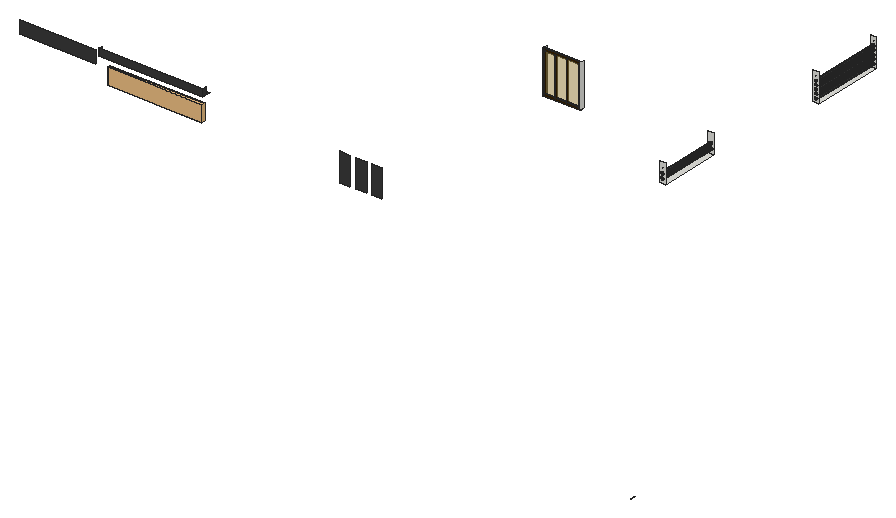
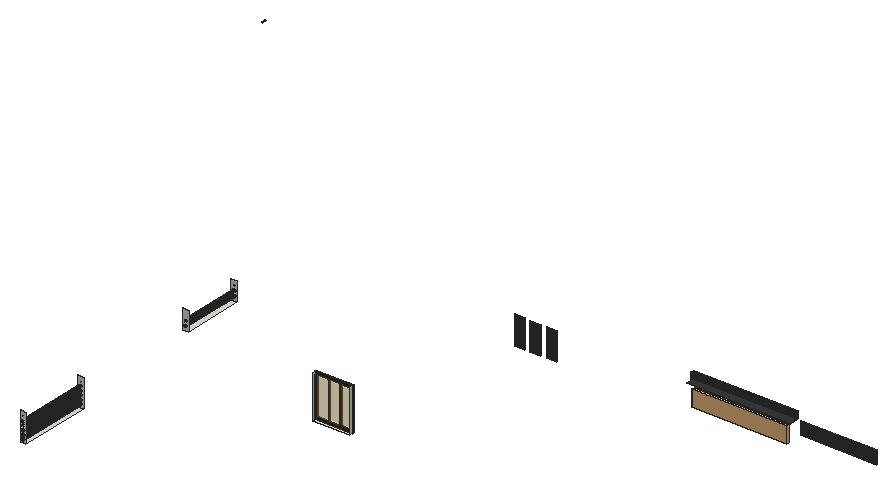
# SketchUp Ruby script. Lengths in inches.
U = 1.inch
M = Sketchup.active_model
def pt(a) = Geom::Point3d.new(a.map { |v| v * U })
def face(e, loops, mat)
  f = e.add_face(loops[0].map { |a| pt(a) })
  loops[1..].each { |l| e.add_face(l.map { |a| pt(a) }).erase! }
  f.material = f.back_material = mat if mat
  f
end
# faces: each face lists its corners as indices into pts; further lists are holes
def faces(e, pts, list, mat = nil) = list.each { |f| face(e, (f[0].is_a?(Array) ? f : [f]).map { |l| l.map { |i| pts[i] } }, mat) }
# xy, xz, yz: faces in a plane at the given z, y or x. An outline is a flat list of corners, or four numbers for a rectangle; further outlines are holes
def ring(l) = l.size == 4 ? [[l[0], l[1]], [l[2], l[1]], [l[2], l[3]], [l[0], l[3]]] : l.each_slice(2).to_a
def flat(e, list, mat, &to3) = list.each { |f| face(e, (f[0].is_a?(Array) ? f : [f]).map { |l| ring(l).map { |u, v| to3.(u, v) } }, mat) }
def xy(e, z, list, mat = nil) = flat(e, list, mat) { |x, y| [x, y, z] }
def xz(e, y, list, mat = nil) = flat(e, list, mat) { |x, z| [x, y, z] }
def yz(e, x, list, mat = nil) = flat(e, list, mat) { |y, z| [x, y, z] }
def lines(e, pts, list) = list.each { |a, b| e.add_line(pt(pts[a]), pt(pts[b])) }
# prism: a flat outline (further loops are holes) pulled along v
def prism(e, loops, v, mat = nil)
  f = face(e, loops, mat); d = Geom::Vector3d.new(v.map { |x| x * U })
  f.pushpull(f.normal.samedirection?(d) ? d.length : -d.length)
end
def box(e, o, s, mat = nil) = prism(e, [[o, [o[0] + s[0], o[1], o[2]], [o[0] + s[0], o[1] + s[1], o[2]], [o[0], o[1] + s[1], o[2]]]], [0, 0, s[2]], mat)
def at(x, y, z, deg = 0) = Geom::Transformation.translation(pt([x, y, z])) * Geom::Transformation.rotation(ORIGIN, Z_AXIS, deg.degrees)
def axes(o, x, y, z) = Geom::Transformation.new([*x, 0, *y, 0, *z, 0, *pt(o).to_a, 1])
def part(name) = M.definitions.add(name)
# library, detail: a bought-in or finely detailed component or shape, given as its bounding box
def library(name, o, s) = part(name).tap { |d| box(d.entities, o, s) }
def detail(e, o, s) = box(e.add_group.entities, o, s)
def put(e, d, t, mat = nil) = e.add_instance(d, t).tap { |i| i.material = mat if mat }
def group(e, t, mat = nil) = e.add_group.tap { |g| g.transformation = t; g.material = mat if mat }.entities
root = M.entities
M.materials.add("[Color A08]").color = [56, 34, 0]
M.materials.add("[Color M07]").color = [58, 58, 58]
M.materials.add("[Color M08]").color = [30, 30, 30]
M.materials.add("[Translucent Glass Blue]").color = [179, 149, 61]
M.materials["[Translucent Glass Blue]"].alpha = 0.5
c1 = part("Group\#2")
xy(c1.entities,0,[[0,0,80.25,5.625]],"[Color A08]")
xy(c1.entities,3.1,[[3.1,0,25.78,5.625],[27.03,0,50.28,5.625],[51.53,0,77.15,5.625]],"[Color A08]")
xy(c1.entities,66.65,[[3.1,0,25.78,5.625],[27.03,0,50.28,5.625],[51.53,0,77.15,5.625]],"[Color A08]")
xy(c1.entities,69.75,[[0,0,80.25,5.625]],"[Color A08]")
xz(c1.entities,0,[[[0,0,80.25,69.75],[51.53,3.1,77.15,66.65],[27.03,3.1,50.28,66.65],[3.1,3.1,25.78,66.65]]],"[Color A08]")
xz(c1.entities,5.625,[[[0,0,80.25,69.75],[51.53,3.1,77.15,66.65],[27.03,3.1,50.28,66.65],[3.1,3.1,25.78,66.65]]],"[Color A08]")
xz(c1.entities,5.625,[[3.1,3.1,25.78,66.65],[27.03,3.1,50.28,66.65],[51.53,3.1,77.15,66.65]],"[Translucent Glass Blue]")
yz(c1.entities,0,[[0,0,5.625,69.75]],"[Color A08]")
yz(c1.entities,3.1,[[0,3.1,5.625,66.65]],"[Color A08]")
yz(c1.entities,25.78,[[0,3.1,5.625,66.65]],"[Color A08]")
yz(c1.entities,27.03,[[0,3.1,5.625,66.65]],"[Color A08]")
yz(c1.entities,50.28,[[0,3.1,5.625,66.65]],"[Color A08]")
yz(c1.entities,51.53,[[0,3.1,5.625,66.65]],"[Color A08]")
yz(c1.entities,77.15,[[0,3.1,5.625,66.65]],"[Color A08]")
yz(c1.entities,80.25,[[0,0,5.625,69.75]],"[Color A08]")
c2 = library("Housedekho",[0.59,0,0],[171.25,24.51,4])
xy(root,58.07,[[560.85,700.96,616.42,706.96]])
xy(root,64.65,[[1254.01,0,1254.88,6]],"[Color M08]")
xy(root,70.51,[[831,872.22,840,980.28]])
xy(root,88.15,[[831,582.45,840,674.33]])
xy(root,94.09,[[132.5,398.15,288.93,411.21]],"[Color M07]")
xz(root,398.15,[[132.5,94.09,288.93,105]],"[Color M07]")
xz(root,402.9,[[491.76,47.23,507.7,89.6],[516.07,47.23,532.01,89.6],[540.01,47.23,555.95,89.6],[9.54,78.4,123.17,97.78]],"[Color M07]")
xz(root,582.45,[[[831,88.15,840,117.03],[835.26,93.06,835.76,93.07,836.25,93.21,836.68,93.48,837.03,93.84,837.27,94.29,837.39,94.78,837.38,95.28,837.23,95.77,836.97,96.2,836.61,96.55,836.16,96.79,835.67,96.91,835.16,96.9,834.68,96.76,834.25,96.49,833.9,96.13,833.66,95.68,833.54,95.19,833.55,94.6875,833.69,94.2,833.95,93.77,834.32,93.42,834.76,93.18],[835.13,100,835.64,100.01,836.12,100.15,836.55,100.41,836.9,100.78,837.14,101.22,837.26,101.71,837.25,102.22,837.11,102.71,836.85,103.14,836.48,103.49,836.04,103.73,835.55,103.85,835.04,103.84,834.55,103.69,834.12,103.43,833.77,103.06,833.53,102.62,833.41,102.13,833.42,101.625,833.57,101.14,833.83,100.71,834.19,100.36,834.64,100.11],[835.13,107.31,835.64,107.32,836.12,107.46,836.55,107.73,836.9,108.09,837.14,108.54,837.26,109.03,837.25,109.53,837.11,110.02,836.85,110.45,836.48,110.8,836.04,111.04,835.55,111.16,835.04,111.15,834.55,111.01,834.12,110.74,833.77,110.38,833.53,109.93,833.41,109.44,833.42,108.9375,833.57,108.45,833.83,108.02,834.19,107.67,834.64,107.43]]])
xz(root,582.45,[[835.26,93.06,835.76,93.07,836.25,93.21,836.68,93.48,837.03,93.84,837.27,94.29,837.39,94.78,837.38,95.28,837.23,95.77,836.97,96.2,836.61,96.55,836.16,96.79,835.67,96.91,835.16,96.9,834.68,96.76,834.25,96.49,833.9,96.13,833.66,95.68,833.54,95.19,833.55,94.6875,833.69,94.2,833.95,93.77,834.32,93.42,834.76,93.18],[835.13,100,835.64,100.01,836.12,100.15,836.55,100.41,836.9,100.78,837.14,101.22,837.26,101.71,837.25,102.22,837.11,102.71,836.85,103.14,836.48,103.49,836.04,103.73,835.55,103.85,835.04,103.84,834.55,103.69,834.12,103.43,833.77,103.06,833.53,102.62,833.41,102.13,833.42,101.625,833.57,101.14,833.83,100.71,834.19,100.36,834.64,100.11]],"[Color M07]")
xz(root,674.14,[[835.13,100,834.64,100.11,834.19,100.36,833.83,100.71,833.57,101.14,833.42,101.625,833.41,102.13,833.53,102.62,833.77,103.06,834.12,103.43,834.55,103.69,835.04,103.84,835.55,103.85,836.04,103.73,836.48,103.49,836.85,103.14,837.11,102.71,837.25,102.22,837.26,101.71,837.14,101.22,836.9,100.78,836.55,100.41,836.12,100.15,835.64,100.01]],"[Color M07]")
xz(root,674.2,[[835.26,93.06,834.76,93.18,834.32,93.42,833.95,93.77,833.69,94.2,833.55,94.6875,833.54,95.19,833.66,95.68,833.9,96.13,834.25,96.49,834.68,96.76,835.16,96.9,835.67,96.91,836.16,96.79,836.61,96.55,836.97,96.2,837.23,95.77,837.38,95.28,837.39,94.78,837.27,94.29,837.03,93.84,836.68,93.48,836.25,93.21,835.76,93.07]],"[Color M07]")
xz(root,674.33,[[831,88.15,840,117.03]])
xz(root,872.22,[[[831,70.51,840,113.38],[835.68,80.13,836.15,80.18,836.59,80.36,836.97,80.64,837.27,81.01,837.45,81.44,837.53,81.91,837.47,82.38,837.3,82.82,837.02,83.2,836.65,83.49,836.21,83.68,835.75,83.75,835.28,83.7,834.84,83.53,834.46,83.25,834.16,82.88,833.97,82.44,833.9,81.98,833.95,81.51,834.125,81.07,834.41,80.68,834.78,80.39,835.21,80.2],[835.68,86.19,836.15,86.25,836.59,86.42,836.97,86.7,837.27,87.07,837.45,87.5,837.53,87.97,837.47,88.44,837.3,88.88,837.02,89.26,836.65,89.56,836.21,89.75,835.75,89.82,835.28,89.76,834.84,89.59,834.46,89.31,834.16,88.94,833.97,88.51,833.9,88.04,833.95,87.57,834.125,87.13,834.41,86.75,834.78,86.45,835.21,86.26],[835.68,92.25,836.15,92.31,836.59,92.48,836.97,92.76,837.27,93.13,837.45,93.57,837.53,94.03,837.47,94.5,837.3,94.94,837.02,95.32,836.65,95.62,836.21,95.81,835.75,95.88,835.28,95.83,834.84,95.65,834.46,95.37,834.16,95,833.97,94.57,833.9,94.1,833.95,93.63,834.125,93.19,834.41,92.81,834.78,92.51,835.21,92.33],[835.68,98.32,836.15,98.37,836.59,98.54,836.97,98.82,837.27,99.19,837.45,99.63,837.53,100.1,837.47,100.57,837.3,101.01,837.02,101.39,836.65,101.68,836.21,101.87,835.75,101.94,835.28,101.89,834.84,101.72,834.46,101.43,834.16,101.06,833.97,100.63,833.9,100.16,833.95,99.69,834.125,99.25,834.41,98.87,834.78,98.58,835.21,98.39],[835.68,104.38,836.15,104.43,836.59,104.61,836.97,104.89,837.27,105.26,837.45,105.69,837.53,106.16,837.47,106.63,837.3,107.07,837.02,107.45,836.65,107.74,836.21,107.93,835.75,108,835.28,107.95,834.84,107.78,834.46,107.5,834.16,107.13,833.97,106.69,833.9,106.23,833.95,105.76,834.125,105.32,834.41,104.93,834.78,104.64,835.21,104.45],[835.68,74.07,836.15,74.12,836.59,74.29,836.97,74.57,837.27,74.94,837.45,75.38,837.53,75.85,837.47,76.32,837.3,76.76,837.02,77.14,836.65,77.43,836.21,77.62,835.75,77.69,835.28,77.64,834.84,77.47,834.46,77.18,834.16,76.81,833.97,76.38,833.9,75.91,833.95,75.44,834.125,75,834.41,74.62,834.78,74.33,835.21,74.14]]])
xz(root,872.22,[[835.68,74.07,836.15,74.12,836.59,74.29,836.97,74.57,837.27,74.94,837.45,75.38,837.53,75.85,837.47,76.32,837.3,76.76,837.02,77.14,836.65,77.43,836.21,77.62,835.75,77.69,835.28,77.64,834.84,77.47,834.46,77.18,834.16,76.81,833.97,76.38,833.9,75.91,833.95,75.44,834.125,75,834.41,74.62,834.78,74.33,835.21,74.14],[835.68,80.13,836.15,80.18,836.59,80.36,836.97,80.64,837.27,81.01,837.45,81.44,837.53,81.91,837.47,82.38,837.3,82.82,837.02,83.2,836.65,83.49,836.21,83.68,835.75,83.75,835.28,83.7,834.84,83.53,834.46,83.25,834.16,82.88,833.97,82.44,833.9,81.98,833.95,81.51,834.125,81.07,834.41,80.68,834.78,80.39,835.21,80.2],[835.68,86.19,836.15,86.25,836.59,86.42,836.97,86.7,837.27,87.07,837.45,87.5,837.53,87.97,837.47,88.44,837.3,88.88,837.02,89.26,836.65,89.56,836.21,89.75,835.75,89.82,835.28,89.76,834.84,89.59,834.46,89.31,834.16,88.94,833.97,88.51,833.9,88.04,833.95,87.57,834.125,87.13,834.41,86.75,834.78,86.45,835.21,86.26],[835.68,92.25,836.15,92.31,836.59,92.48,836.97,92.76,837.27,93.13,837.45,93.57,837.53,94.03,837.47,94.5,837.3,94.94,837.02,95.32,836.65,95.62,836.21,95.81,835.75,95.88,835.28,95.83,834.84,95.65,834.46,95.37,834.16,95,833.97,94.57,833.9,94.1,833.95,93.63,834.125,93.19,834.41,92.81,834.78,92.51,835.21,92.33],[835.68,98.32,836.15,98.37,836.59,98.54,836.97,98.82,837.27,99.19,837.45,99.63,837.53,100.1,837.47,100.57,837.3,101.01,837.02,101.39,836.65,101.68,836.21,101.87,835.75,101.94,835.28,101.89,834.84,101.72,834.46,101.43,834.16,101.06,833.97,100.63,833.9,100.16,833.95,99.69,834.125,99.25,834.41,98.87,834.78,98.58,835.21,98.39]],"[Color M07]")
xz(root,980.03,[[835.68,92.25,835.21,92.33,834.78,92.51,834.41,92.81,834.125,93.19,833.95,93.63,833.9,94.1,833.97,94.57,834.16,95,834.46,95.37,834.84,95.65,835.28,95.83,835.75,95.88,836.21,95.81,836.65,95.62,837.02,95.32,837.3,94.94,837.47,94.5,837.53,94.03,837.45,93.57,837.27,93.13,836.97,92.76,836.59,92.48,836.15,92.31],[835.68,98.32,835.21,98.39,834.78,98.58,834.41,98.87,834.125,99.25,833.95,99.69,833.9,100.16,833.97,100.63,834.16,101.06,834.46,101.43,834.84,101.72,835.28,101.89,835.75,101.94,836.21,101.87,836.65,101.68,837.02,101.39,837.3,101.01,837.47,100.57,837.53,100.1,837.45,99.63,837.27,99.19,836.97,98.82,836.59,98.54,836.15,98.37]],"[Color M07]")
xz(root,980.28,[[[831,70.51,840,113.38],[835.68,86.19,835.21,86.26,834.78,86.45,834.41,86.75,834.125,87.13,833.95,87.57,833.9,88.04,833.97,88.51,834.16,88.94,834.46,89.31,834.84,89.59,835.28,89.76,835.75,89.82,836.21,89.75,836.65,89.56,837.02,89.26,837.3,88.88,837.47,88.44,837.53,87.97,837.45,87.5,837.27,87.07,836.97,86.7,836.59,86.42,836.15,86.25],[835.68,104.38,835.21,104.45,834.78,104.64,834.41,104.93,834.125,105.32,833.95,105.76,833.9,106.23,833.97,106.69,834.16,107.13,834.46,107.5,834.84,107.78,835.28,107.95,835.75,108,836.21,107.93,836.65,107.74,837.02,107.45,837.3,107.07,837.47,106.63,837.53,106.16,837.45,105.69,837.27,105.26,836.97,104.89,836.59,104.61,836.15,104.43]]])
xz(root,980.34,[[835.68,74.07,835.21,74.14,834.78,74.33,834.41,74.62,834.125,75,833.95,75.44,833.9,75.91,833.97,76.38,834.16,76.81,834.46,77.18,834.84,77.47,835.28,77.64,835.75,77.69,836.21,77.62,836.65,77.43,837.02,77.14,837.3,76.76,837.47,76.32,837.53,75.85,837.45,75.38,837.27,74.94,836.97,74.57,836.59,74.29,836.15,74.12]],"[Color M07]")
xz(root,981.09,[[835.68,80.13,835.21,80.2,834.78,80.39,834.41,80.68,834.125,81.07,833.95,81.51,833.9,81.98,833.97,82.44,834.16,82.88,834.46,83.25,834.84,83.53,835.28,83.7,835.75,83.75,836.21,83.68,836.65,83.49,837.02,83.2,837.3,82.82,837.47,82.38,837.53,81.91,837.45,81.44,837.27,81.01,836.97,80.64,836.59,80.36,836.15,80.18]],"[Color M07]")
yz(root,132.5,[[398.15,94.09,402.9,105]],"[Color M07]")
yz(root,288.93,[[398.15,94.09,402.9,105]],"[Color M07]")
yz(root,560.85,[[700.96,58.07,706.96,122.82]])
yz(root,616.42,[[700.96,58.07,706.96,122.82]])
p = [[835.21,872.22,74.14],[834.78,872.22,74.33],[834.78,980.34,74.33],[835.21,980.34,74.14],[835.68,872.22,74.07],[835.68,980.34,74.07],
  [836.15,872.22,74.12],[836.15,980.34,74.12],[836.59,872.22,74.29],[836.59,980.34,74.29],[834.41,872.22,74.62],[834.41,980.34,74.62],
  [836.97,872.22,74.57],[836.97,980.34,74.57],[834.125,872.22,75],[834.125,980.34,75],[837.27,872.22,74.94],[837.27,980.34,74.94],
  [837.45,872.22,75.38],[837.45,980.34,75.38],[833.95,872.22,75.44],[833.95,980.34,75.44],[833.9,872.22,75.91],[833.9,980.34,75.91],
  [837.53,872.22,75.85],[837.53,980.34,75.85],[837.47,872.22,76.32],[837.47,980.34,76.32],[833.97,872.22,76.38],[833.97,980.34,76.38],
  [837.3,872.22,76.76],[837.3,980.34,76.76],[834.16,872.22,76.81],[834.16,980.34,76.81],[834.46,872.22,77.18],[834.46,980.34,77.18],
  [837.02,872.22,77.14],[837.02,980.34,77.14],[836.65,872.22,77.43],[836.65,980.34,77.43],[834.84,872.22,77.47],[834.84,980.34,77.47],
  [836.21,872.22,77.62],[836.21,980.34,77.62],[835.28,872.22,77.64],[835.28,980.34,77.64],[835.75,872.22,77.69],[835.75,980.34,77.69],
  [835.68,872.22,80.13],[835.21,872.22,80.2],[835.21,981.09,80.2],[835.68,981.09,80.13],[836.15,872.22,80.18],[836.15,981.09,80.18],
  [834.78,872.22,80.39],[834.78,981.09,80.39],[836.59,872.22,80.36],[836.59,981.09,80.36],[834.41,872.22,80.68],[834.41,981.09,80.68],
  [836.97,872.22,80.64],[836.97,981.09,80.64],[837.27,872.22,81.01],[837.27,981.09,81.01],[834.125,872.22,81.07],[834.125,981.09,81.07],
  [837.45,872.22,81.44],[837.45,981.09,81.44],[833.95,872.22,81.51],[833.95,981.09,81.51],[837.53,872.22,81.91],[837.53,981.09,81.91],
  [833.9,872.22,81.98],[833.9,981.09,81.98],[837.47,872.22,82.38],[837.47,981.09,82.38],[833.97,872.22,82.44],[833.97,981.09,82.44],
  [834.16,872.22,82.88],[834.16,981.09,82.88],[837.3,872.22,82.82],[837.3,981.09,82.82],[837.02,872.22,83.2],[837.02,981.09,83.2],
  [834.46,872.22,83.25],[834.46,981.09,83.25],[834.84,872.22,83.53],[834.84,981.09,83.53],[836.65,872.22,83.49],[836.65,981.09,83.49],
  [835.28,872.22,83.7],[835.28,981.09,83.7],[836.21,872.22,83.68],[836.21,981.09,83.68],[835.75,872.22,83.75],[835.75,981.09,83.75],
  [835.68,872.22,86.19],[835.21,872.22,86.26],[835.21,980.28,86.26],[835.68,980.28,86.19],[836.15,872.22,86.25],[836.15,980.28,86.25],
  [836.59,872.22,86.42],[836.59,980.28,86.42],[834.78,872.22,86.45],[834.78,980.28,86.45],[836.97,872.22,86.7],[836.97,980.28,86.7],
  [834.41,872.22,86.75],[834.41,980.28,86.75],[834.125,872.22,87.13],[834.125,980.28,87.13],[837.27,872.22,87.07],[837.27,980.28,87.07],
  [833.95,872.22,87.57],[833.95,980.28,87.57],[837.45,872.22,87.5],[837.45,980.28,87.5],[837.53,872.22,87.97],[837.53,980.28,87.97],
  [833.9,872.22,88.04],[833.9,980.28,88.04],[833.97,872.22,88.51],[833.97,980.28,88.51],[837.47,872.22,88.44],[837.47,980.28,88.44],
  [837.3,872.22,88.88],[837.3,980.28,88.88],[834.16,872.22,88.94],[834.16,980.28,88.94],[834.46,872.22,89.31],[834.46,980.28,89.31],
  [837.02,872.22,89.26],[837.02,980.28,89.26],[834.84,872.22,89.59],[834.84,980.28,89.59],[836.65,872.22,89.56],[836.65,980.28,89.56],
  [835.28,872.22,89.76],[835.28,980.28,89.76],[836.21,872.22,89.75],[836.21,980.28,89.75],[835.75,872.22,89.82],[835.75,980.28,89.82],
  [835.21,872.22,92.33],[834.78,872.22,92.51],[834.78,980.03,92.51],[835.21,980.03,92.33],[835.68,872.22,92.25],[835.68,980.03,92.25],
  [836.15,872.22,92.31],[836.15,980.03,92.31],[836.59,872.22,92.48],[836.59,980.03,92.48],[834.41,872.22,92.81],[834.41,980.03,92.81],
  [836.97,872.22,92.76],[836.97,980.03,92.76],[834.125,872.22,93.19],[834.125,980.03,93.19],[837.27,872.22,93.13],[837.27,980.03,93.13],
  [835.26,582.45,93.06],[834.76,582.45,93.18],[834.76,674.2,93.18],[835.26,674.2,93.06],[835.76,582.45,93.07],[835.76,674.2,93.07],
  [836.25,582.45,93.21],[836.25,674.2,93.21],[837.45,872.22,93.57],[837.45,980.03,93.57],[834.32,582.45,93.42],[834.32,674.2,93.42],
  [836.68,582.45,93.48],[836.68,674.2,93.48],[833.95,872.22,93.63],[833.95,980.03,93.63],[833.95,582.45,93.77],[833.95,674.2,93.77],
  [837.03,582.45,93.84],[837.03,674.2,93.84],[833.9,872.22,94.1],[833.9,980.03,94.1],[837.53,872.22,94.03],[837.53,980.03,94.03],
  [833.69,582.45,94.2],[833.69,674.2,94.2],[837.27,582.45,94.29],[837.27,674.2,94.29],[837.47,872.22,94.5],[837.47,980.03,94.5],
  [833.97,872.22,94.57],[833.97,980.03,94.57],[833.55,582.45,94.6875],[833.55,674.2,94.6875],[837.39,582.45,94.78],[837.39,674.2,94.78],
  [837.3,872.22,94.94],[837.3,980.03,94.94],[834.16,872.22,95],[834.16,980.03,95],[833.54,582.45,95.19],[833.54,674.2,95.19],
  [837.38,582.45,95.28],[837.38,674.2,95.28],[837.02,872.22,95.32],[837.02,980.03,95.32],[834.46,872.22,95.37],[834.46,980.03,95.37],
  [833.66,582.45,95.68],[833.66,674.2,95.68],[837.23,582.45,95.77],[837.23,674.2,95.77],[836.65,872.22,95.62],[836.65,980.03,95.62],
  [834.84,872.22,95.65],[834.84,980.03,95.65],[836.21,872.22,95.81],[836.21,980.03,95.81],[833.9,582.45,96.13],[833.9,674.2,96.13],
  [835.28,872.22,95.83],[835.28,980.03,95.83],[836.97,582.45,96.2],[836.97,674.2,96.2],[835.75,872.22,95.88],[835.75,980.03,95.88],
  [834.25,582.45,96.49],[834.25,674.2,96.49],[836.61,582.45,96.55],[836.61,674.2,96.55],[834.68,582.45,96.76],[834.68,674.2,96.76],
  [836.16,582.45,96.79],[836.16,674.2,96.79],[835.16,582.45,96.9],[835.16,674.2,96.9],[835.67,582.45,96.91],[835.67,674.2,96.91],
  [835.68,872.22,98.32],[835.21,872.22,98.39],[835.21,980.03,98.39],[835.68,980.03,98.32],[836.15,872.22,98.37],[836.15,980.03,98.37],
  [834.78,872.22,98.58],[834.78,980.03,98.58],[836.59,872.22,98.54],[836.59,980.03,98.54],[836.97,872.22,98.82],[836.97,980.03,98.82],
  [834.41,872.22,98.87],[834.41,980.03,98.87],[837.27,872.22,99.19],[837.27,980.03,99.19],[834.125,872.22,99.25],[834.125,980.03,99.25],
  [837.45,872.22,99.63],[837.45,980.03,99.63],[833.95,872.22,99.69],[833.95,980.03,99.69],[837.53,872.22,100.1],[837.53,980.03,100.1],
  [833.9,872.22,100.16],[833.9,980.03,100.16],[835.13,582.45,100],[834.64,582.45,100.11],[834.64,674.14,100.11],[835.13,674.14,100],
  [835.64,582.45,100.01],[835.64,674.14,100.01],[836.12,582.45,100.15],[836.12,674.14,100.15],[834.19,582.45,100.36],[834.19,674.14,100.36],
  [836.55,582.45,100.41],[836.55,674.14,100.41],[837.47,872.22,100.57],[837.47,980.03,100.57],[833.97,872.22,100.63],[833.97,980.03,100.63],
  [833.83,582.45,100.71],[833.83,674.14,100.71],[836.9,582.45,100.78],[836.9,674.14,100.78],[834.16,872.22,101.06],[834.16,980.03,101.06],
  [837.3,872.22,101.01],[837.3,980.03,101.01],[833.57,582.45,101.14],[833.57,674.14,101.14],[837.14,582.45,101.22],[837.14,674.14,101.22],
  [837.02,872.22,101.39],[837.02,980.03,101.39],[833.42,582.45,101.625],[833.42,674.14,101.625],[834.46,872.22,101.43],[834.46,980.03,101.43],
  [837.26,582.45,101.71],[837.26,674.14,101.71],[834.84,872.22,101.72],[834.84,980.03,101.72],[836.65,872.22,101.68],[836.65,980.03,101.68],
  [833.41,582.45,102.13],[833.41,674.14,102.13],[837.25,582.45,102.22],[837.25,674.14,102.22],[835.28,872.22,101.89],[835.28,980.03,101.89],
  [836.21,872.22,101.87],[836.21,980.03,101.87],[835.75,872.22,101.94],[835.75,980.03,101.94],[833.53,582.45,102.62],[833.53,674.14,102.62],
  [837.11,582.45,102.71],[837.11,674.14,102.71],[833.77,582.45,103.06],[833.77,674.14,103.06],[836.85,582.45,103.14],[836.85,674.14,103.14],
  [834.12,582.45,103.43],[834.12,674.14,103.43],[836.48,582.45,103.49],[836.48,674.14,103.49],[834.55,582.45,103.69],[834.55,674.14,103.69],
  [836.04,582.45,103.73],[836.04,674.14,103.73],[835.04,582.45,103.84],[835.04,674.14,103.84],[835.55,582.45,103.85],[835.55,674.14,103.85]]
faces(root,p,[[0,1,2,3],[4,0,3,5],[6,4,5,7],[8,6,7,9],[1,10,11,2],[12,8,9,13],[10,14,15,11],[16,12,13,17],
  [18,16,17,19],[14,20,21,15],[20,22,23,21],[24,18,19,25],[26,24,25,27],[22,28,29,23],[30,26,27,31],[28,32,33,29],
  [32,34,35,33],[36,30,31,37],[38,36,37,39],[34,40,41,35],[42,38,39,43],[40,44,45,41],[44,46,47,45],[46,42,43,47],
  [48,49,50,51],[52,48,51,53],[49,54,55,50],[56,52,53,57],[54,58,59,55],[60,56,57,61],[62,60,61,63],[58,64,65,59],
  [66,62,63,67],[64,68,69,65],[70,66,67,71],[68,72,73,69],[74,70,71,75],[72,76,77,73],[76,78,79,77],[80,74,75,81],
  [82,80,81,83],[78,84,85,79],[84,86,87,85],[88,82,83,89],[86,90,91,87],[92,88,89,93],[90,94,95,91],[94,92,93,95],
  [96,97,98,99],[100,96,99,101],[102,100,101,103],[97,104,105,98],[106,102,103,107],[104,108,109,105],[108,110,111,109],[112,106,107,113],
  [110,114,115,111],[116,112,113,117],[118,116,117,119],[114,120,121,115],[120,122,123,121],[124,118,119,125],[126,124,125,127],[122,128,129,123],
  [128,130,131,129],[132,126,127,133],[130,134,135,131],[136,132,133,137],[134,138,139,135],[140,136,137,141],[142,140,141,143],[138,142,143,139],
  [144,145,146,147],[148,144,147,149],[150,148,149,151],[152,150,151,153],[145,154,155,146],[156,152,153,157],[154,158,159,155],[160,156,157,161],
  [162,163,164,165],[166,162,165,167],[168,166,167,169],[170,160,161,171],[163,172,173,164],[174,168,169,175],[158,176,177,159],[172,178,179,173],
  [180,174,175,181],[176,182,183,177],[184,170,171,185],[178,186,187,179],[188,180,181,189],[190,184,185,191],[182,192,193,183],[186,194,195,187],
  [196,188,189,197],[198,190,191,199],[192,200,201,193],[194,202,203,195],[204,196,197,205],[206,198,199,207],[200,208,209,201],[202,210,211,203],
  [212,204,205,213],[214,206,207,215],[208,216,217,209],[218,214,215,219],[210,220,221,211],[216,222,223,217],[224,212,213,225],[222,226,227,223],
  [226,218,219,227],[220,228,229,221],[230,224,225,231],[228,232,233,229],[234,230,231,235],[232,236,237,233],[238,234,235,239],[236,238,239,237],
  [240,241,242,243],[244,240,243,245],[241,246,247,242],[248,244,245,249],[250,248,249,251],[246,252,253,247],[254,250,251,255],[252,256,257,253],
  [258,254,255,259],[256,260,261,257],[262,258,259,263],[260,264,265,261],[266,267,268,269],[270,266,269,271],[272,270,271,273],[267,274,275,268],
  [276,272,273,277],[278,262,263,279],[264,280,281,265],[274,282,283,275],[284,276,277,285],[280,286,287,281],[288,278,279,289],[282,290,291,283],
  [292,284,285,293],[294,288,289,295],[290,296,297,291],[286,298,299,287],[300,292,293,301],[298,302,303,299],[304,294,295,305],[296,306,307,297],
  [308,300,301,309],[302,310,311,303],[312,304,305,313],[310,314,315,311],[314,312,313,315],[306,316,317,307],[318,308,309,319],[316,320,321,317],
  [322,318,319,323],[320,324,325,321],[326,322,323,327],[324,328,329,325],[330,326,327,331],[328,332,333,329],[334,330,331,335],[332,334,335,333]],"[Color M07]")
put(root,c1,axes([560.3,700.96,58.07],[0.6993,0,0],[0,0.37,0],[0,0,0.92832]))
put(root,c2,axes([143.6875,402.9,58.49],[0.837,0,0],[0,0,1],[0,-1,0]))
